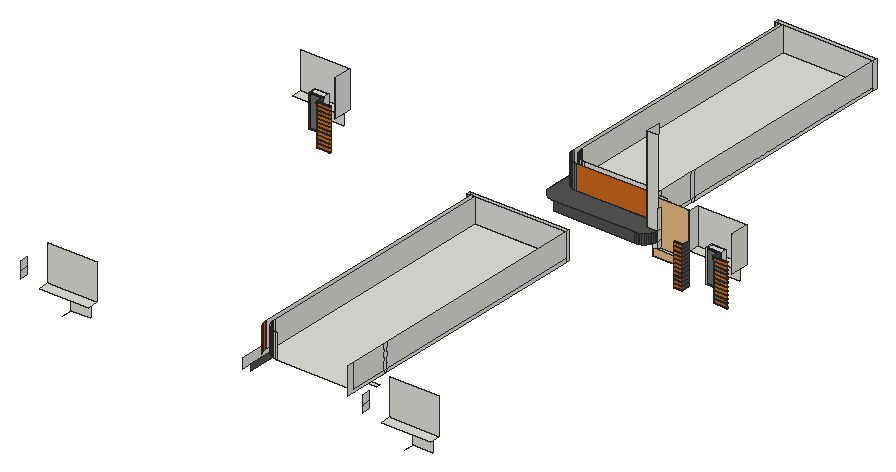
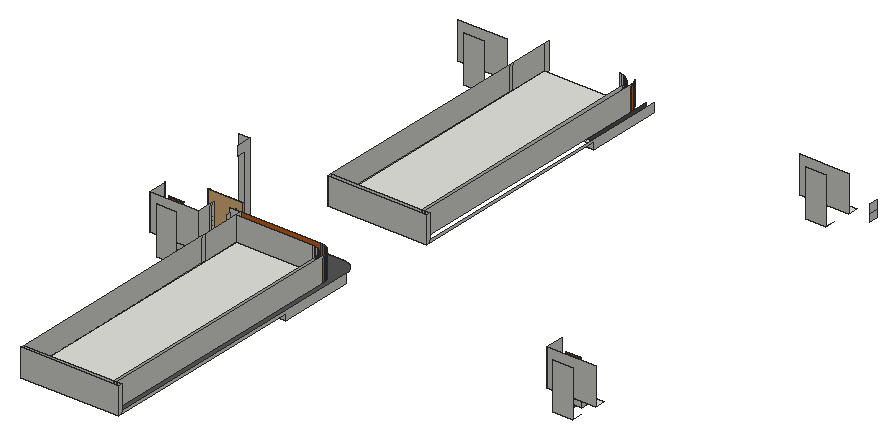
# SketchUp Ruby script. Lengths in inches.
U = 1.inch
M = Sketchup.active_model
def pt(a) = Geom::Point3d.new(a.map { |v| v * U })
def face(e, loops, mat)
  f = e.add_face(loops[0].map { |a| pt(a) })
  loops[1..].each { |l| e.add_face(l.map { |a| pt(a) }).erase! }
  f.material = f.back_material = mat if mat
  f
end
# faces: each face lists its corners as indices into pts; further lists are holes
def faces(e, pts, list, mat = nil) = list.each { |f| face(e, (f[0].is_a?(Array) ? f : [f]).map { |l| l.map { |i| pts[i] } }, mat) }
# xy, xz, yz: faces in a plane at the given z, y or x. An outline is a flat list of corners, or four numbers for a rectangle; further outlines are holes
def ring(l) = l.size == 4 ? [[l[0], l[1]], [l[2], l[1]], [l[2], l[3]], [l[0], l[3]]] : l.each_slice(2).to_a
def flat(e, list, mat, &to3) = list.each { |f| face(e, (f[0].is_a?(Array) ? f : [f]).map { |l| ring(l).map { |u, v| to3.(u, v) } }, mat) }
def xy(e, z, list, mat = nil) = flat(e, list, mat) { |x, y| [x, y, z] }
def xz(e, y, list, mat = nil) = flat(e, list, mat) { |x, z| [x, y, z] }
def yz(e, x, list, mat = nil) = flat(e, list, mat) { |y, z| [x, y, z] }
def lines(e, pts, list) = list.each { |a, b| e.add_line(pt(pts[a]), pt(pts[b])) }
# prism: a flat outline (further loops are holes) pulled along v
def prism(e, loops, v, mat = nil)
  f = face(e, loops, mat); d = Geom::Vector3d.new(v.map { |x| x * U })
  f.pushpull(f.normal.samedirection?(d) ? d.length : -d.length)
end
def box(e, o, s, mat = nil) = prism(e, [[o, [o[0] + s[0], o[1], o[2]], [o[0] + s[0], o[1] + s[1], o[2]], [o[0], o[1] + s[1], o[2]]]], [0, 0, s[2]], mat)
def at(x, y, z, deg = 0) = Geom::Transformation.translation(pt([x, y, z])) * Geom::Transformation.rotation(ORIGIN, Z_AXIS, deg.degrees)
def axes(o, x, y, z) = Geom::Transformation.new([*x, 0, *y, 0, *z, 0, *pt(o).to_a, 1])
def part(name) = M.definitions.add(name)
# library, detail: a bought-in or finely detailed component or shape, given as its bounding box
def library(name, o, s) = part(name).tap { |d| box(d.entities, o, s) }
def detail(e, o, s) = box(e.add_group.entities, o, s)
def put(e, d, t, mat = nil) = e.add_instance(d, t).tap { |i| i.material = mat if mat }
def group(e, t, mat = nil) = e.add_group.tap { |g| g.transformation = t; g.material = mat if mat }.entities
root = M.entities
M.materials.add("[0039_DarkOrange]").color = [219, 120, 0]
M.materials.add("[0041_Chocolate]").color = [210, 105, 30]
M.materials.add("[Color M06]").color = [84, 84, 84]
M.materials.add("[Translucent Glass Gray]").color = [0, 0, 0]
M.materials["[Translucent Glass Gray]"].alpha = 0.5
c1 = library("1",[3.97,34.78,0],[101.43,33.99,0.79])
xy(root,180.58,[[1550.98,971.36,1577.46,972.36],[2230.65,971.36,2246.03,972.36],[2305.61,971.36,2332.08,972.36]],"[0041_Chocolate]")
xy(root,182.6875,[[1550.98,971.36,1577.46,972.36],[2230.65,971.36,2246.03,972.36],[2305.61,971.36,2332.08,972.36]],"[0041_Chocolate]")
xy(root,187.64,[[1550.98,971.36,1577.46,972.36],[2230.65,971.36,2246.03,972.36],[2305.61,971.36,2332.08,972.36]],"[0041_Chocolate]")
xy(root,189.75,[[1550.98,971.36,1577.46,972.36],[2230.65,971.36,2246.03,972.36],[2305.61,971.36,2332.08,972.36]],"[0041_Chocolate]")
xy(root,194.7,[[1550.98,971.36,1577.46,972.36],[2230.65,971.36,2246.03,972.36],[2305.61,971.36,2332.08,972.36]],"[0041_Chocolate]")
xy(root,196.8125,[[1550.98,971.36,1577.46,972.36],[2305.61,971.36,2332.08,972.36]],"[0039_DarkOrange]")
xy(root,196.8125,[[2230.65,971.36,2246.03,972.36]],"[0041_Chocolate]")
xy(root,196.89,[[1523.64,986.55,1550.33,989.22],[2278.27,986.55,2304.96,989.22],[1523.64,990.13,1550.33,1001.8],[2278.27,990.13,2304.96,1001.8]])
xy(root,201.77,[[1550.98,971.36,1577.46,972.36],[2305.61,971.36,2332.08,972.36]],"[0039_DarkOrange]")
xy(root,201.77,[[2230.65,971.36,2246.03,972.36]],"[0041_Chocolate]")
xy(root,203.875,[[1550.98,971.36,1577.46,972.36],[2305.61,971.36,2332.08,972.36]],"[0039_DarkOrange]")
xy(root,203.875,[[2230.65,971.36,2246.03,972.36]],"[0041_Chocolate]")
xy(root,208.83,[[1550.98,971.36,1577.46,972.36],[2305.61,971.36,2332.08,972.36]],"[0039_DarkOrange]")
xy(root,208.83,[[2230.65,971.36,2246.03,972.36]],"[0041_Chocolate]")
xy(root,210.9375,[[1550.98,971.36,1577.46,972.36],[2305.61,971.36,2332.08,972.36]],"[0039_DarkOrange]")
xy(root,210.9375,[[2230.65,971.36,2246.03,972.36]],"[0041_Chocolate]")
xy(root,215.89,[[1550.98,971.36,1577.46,972.36],[2305.61,971.36,2332.08,972.36]],"[0039_DarkOrange]")
xy(root,215.89,[[2230.65,971.36,2246.03,972.36]],"[0041_Chocolate]")
xy(root,218,[[1550.98,971.36,1577.46,972.36],[2305.61,971.36,2332.08,972.36]],"[0039_DarkOrange]")
xy(root,218,[[2230.65,971.36,2246.03,972.36]],"[0041_Chocolate]")
xy(root,222.95,[[1550.98,971.36,1577.46,972.36],[2305.61,971.36,2332.08,972.36]],"[0039_DarkOrange]")
xy(root,222.95,[[2230.65,971.36,2246.03,972.36]],"[0041_Chocolate]")
xy(root,225.0625,[[1550.98,971.36,1577.46,972.36],[2305.61,971.36,2332.08,972.36]],"[0039_DarkOrange]")
xy(root,225.0625,[[2230.65,971.36,2246.03,972.36]],"[0041_Chocolate]")
xy(root,226.8,[[1547.71,317.3125,1640.52,337.5625],[2198.21,317.3125,2291.02,337.5625],[2181.03,983.34,2190.68,996.48],[2190.68,983.34,2230.65,1028.46],[1476.02,1008.21,1568.84,1028.46],
  [2230.65,1008.21,2323.46,1028.46]])
xy(root,227.53,[[2078.42,395.98,2125.61,403.17],[2110.86,1086.875,2158.05,1094.0625]])
xy(root,230.02,[[1550.98,971.36,1577.46,972.36],[2305.61,971.36,2332.08,972.36]],"[0039_DarkOrange]")
xy(root,230.02,[[2230.65,971.36,2246.03,972.36]],"[0041_Chocolate]")
xy(root,232.125,[[1550.98,971.36,1577.46,972.36],[2305.61,971.36,2332.08,972.36]],"[0039_DarkOrange]")
xy(root,232.125,[[2230.65,971.36,2246.03,972.36]],"[0041_Chocolate]")
xy(root,237.08,[[1550.98,971.36,1577.46,972.36],[2305.61,971.36,2332.08,972.36]],"[0039_DarkOrange]")
xy(root,237.08,[[2230.65,971.36,2246.03,972.36]],"[0041_Chocolate]")
xy(root,239.1875,[[1550.98,971.36,1577.46,972.36],[2230.65,971.36,2246.03,972.36],[2305.61,971.36,2332.08,972.36]],"[0041_Chocolate]")
xy(root,240.16,[[2166.32,969.24,2169.44,972.36],[2166.57,972.36,2167.81,972.44,2169.03,972.69,2169.44,972.82,2169.44,972.36],[2169.44,972.36,2169.44,972.82,2170.21,973.09,2171.33,973.64,2172.37,974.33,2173.31,975.15,2174.13,976.09,2174.82,977.13,2175.375,978.25,2175.77,979.43,2176.02,980.65,2176.1,981.89,2169.44,981.89,2169.44,983.34,2189.82,983.34,2189.82,981.89,2189.62,978.86,2189.02,975.875,2188.05,973,2187.73,972.36],[2187.73,972.36,2190.68,972.36,2190.68,981.89,2189.82,981.89,2189.62,978.86,2189.02,975.875,2188.05,973],[2169.44,972.82,2170.21,973.09,2171.33,973.64,2172.37,974.33,2173.31,975.15,2174.13,976.09,2174.82,977.13,2175.375,978.25,2175.77,979.43,2176.02,980.65,2176.1,981.89,2169.44,981.89],
  [2189.82,981.89,2190.68,983.34],[2169.44,983.34,2189.82,1003.71],[2189.82,983.34,2190.68,1003.71]])
xy(root,240.16,[[1949.9,333.33,1963.61,439.98],[2012.97,958.64,2012.97,972.36,2132.44,972.36,2132.44,969.24,2135.57,969.24,2135.57,972.36,2136.69,972.36,2136.69,969.24,2139.82,969.24,2139.82,972.36,2140.94,972.36,2140.94,969.24,2144.07,969.24,2144.07,972.36,2145.19,972.36,2145.19,969.24,2148.32,969.24,2148.32,972.36,2149.38,972.36,2149.38,969.24,2152.5,969.24,2152.5,972.36,2153.57,972.36,2153.57,969.24,2156.69,969.24,2156.69,972.36,2157.75,972.36,2157.75,969.24,2160.88,969.24,2160.88,972.36,2161.94,972.36,2161.94,969.24,2165.07,969.24,2165.07,972.36,2166.32,972.36,2166.32,969.24,2169.44,969.24,2169.44,972.36,2187.73,972.36,2186.7,970.27,2185.01,967.74,2183.01,965.45,2180.72,963.45,2178.19,961.76,2175.46,960.41,2172.58,959.4375,2169.6,958.84,2166.57,958.64],[1982.33,1024.22,1996.05,1130.875]],"[Color M06]")
xy(root,244.14,[[1550.98,971.36,1577.46,972.36],[2230.65,971.36,2246.03,972.36],[2305.61,971.36,2332.08,972.36]],"[0041_Chocolate]")
xy(root,246.25,[[1550.98,971.36,1577.46,972.36],[2230.65,971.36,2246.03,972.36],[2305.61,971.36,2332.08,972.36]],"[0041_Chocolate]")
xy(root,251.2,[[1550.98,971.36,1577.46,972.36],[2230.65,971.36,2246.03,972.36],[2305.61,971.36,2332.08,972.36]],"[0041_Chocolate]")
xy(root,252.47,[[[2066.68,395.98,2137,395.98,2137,403.17,2084.26,403.17,2084.26,439.98,2137,439.98,2137,830.91,1949.9,830.91,1949.9,439.98,2066.68,439.98],[1955.4,445.49,2131.5,825.41]],[2084.26,403.17,2137,439.98],[1949.9,830.91,2137,838.14],[2012.97,972.36,2010.76,972.5,2008.59,972.9375,2006.5,973.65,2004.51,974.63,2002.67,975.86,2001.01,977.32,1999.55,978.98,1998.32,980.82,1997.34,982.81,1996.625,984.9,1996.2,987.07,1996.05,989.28,1996.05,1130.875,2099.12,1130.875,2099.12,1086.875,2169.44,1086.875,2169.44,981.89,2176.1,981.89,2176.02,980.65,2175.77,979.43,2175.375,978.25,2174.82,977.13,2174.13,976.09,2173.31,975.15,2172.37,974.33,2171.33,973.64,2170.21,973.09,2169.03,972.69,2167.81,972.44,2166.57,972.36],[[2099.12,1086.875,2169.44,1086.875,2169.44,1094.0625,2116.69,1094.0625,2116.69,1130.875,2169.44,1130.875,2169.44,1521.81,1982.33,1521.81,1982.33,1130.875,2099.12,1130.875],[1987.84,1136.38,2163.94,1516.3]],
  [2116.69,1094.0625,2169.44,1130.875],[1982.33,1521.81,2169.44,1529.04]])
xy(root,253.3125,[[1550.98,971.36,1577.46,972.36],[2230.65,971.36,2246.03,972.36],[2305.61,971.36,2332.08,972.36]],"[0041_Chocolate]")
xy(root,258.13,[[1993.24,325.34,2137,325.34,2137,830.91,1965.22,830.91,1965.22,353.36,1965.46,349.7,1966.18,346.11,1967.36,342.64,1968.98,339.35,1971.01,336.3,1973.43,333.55,1976.1875,331.13,1979.23,329.09,1982.52,327.47,1985.99,326.29,1989.59,325.58],[2189.82,983.34,2190.68,1003.71],[2025.68,1016.23,2169.44,1016.23,2169.44,1521.81,1997.66,1521.81,1997.66,1044.25,1997.9,1040.6,1998.62,1037,1999.8,1033.53,2001.42,1030.24,2003.45,1027.2,2005.87,1024.44,2008.625,1022.02,2011.67,1019.99,2014.96,1018.37,2018.43,1017.1875,2022.02,1016.47]])
xy(root,258.13,[[2012.97,958.64,2166.57,958.64,2169.6,958.84,2172.58,959.4375,2175.46,960.41,2178.19,961.76,2180.72,963.45,2183.01,965.45,2185.01,967.74,2186.7,970.27,2188.05,973,2189.02,975.875,2189.62,978.86,2189.82,981.89,2189.82,1003.71,2019.9375,1003.71,2016.14,1003.96,2012.42,1004.7,2008.82,1005.92,2005.41,1007.6,2002.25,1009.71,1999.39,1012.22,1996.88,1015.08,1996.11,1016.23,1994.77,1018.24,1993.09,1021.65,1991.87,1025.25,1991.125,1028.97,1990.88,1032.77,1990.88,1521.81,1982.33,1521.81,1982.33,989.28,1982.6,985.28,1983.38,981.35,1984.67,977.56,1986.4375,973.96,1988.67,970.63,1991.31,967.62,1994.32,964.98,1997.65,962.75,2001.25,960.98,2005.04,959.6875,2008.97,958.91]],"[Color M06]")
xy(root,258.27,[[1523.64,986.55,1550.33,989.22],[2278.27,986.55,2304.96,989.22],[1523.64,989.22,1550.33,990.13],[2278.27,989.22,2304.96,990.13],[1523.64,990.13,1550.33,1001.8],
  [2278.27,990.13,2304.96,1001.8]])
xy(root,258.27,[[1550.33,971.36,1577.46,972.36],[2230.65,971.36,2246.69,972.36],[2304.96,971.36,2332.08,972.36]],"[0041_Chocolate]")
xz(root,337.5625,[[1547.71,226.8,1640.52,295.72],[2198.21,226.8,2291.02,295.72]])
xz(root,341.65,[[1588.08,192.35,1624.95,281.26],[2238.58,192.35,2275.45,281.26]])
xz(root,439.98,[[1949.9,240.16,1963.61,252.47]])
xz(root,830.91,[[1949.9,252.47,1949.9,258.13,1958.44,258.13,1958.44,304.25,1965.22,304.25,1965.22,258.13,2137,258.13,2137,252.47],[1949.9,258.13,1958.44,304.25],[1965.22,258.13,2137,304.25]])
xz(root,838.14,[[1949.9,252.47,2137,304.25]])
xz(root,958.64,[[2012.97,240.16,2166.57,258.13]],"[Color M06]")
xz(root,971.36,[[1550.98,196.8125,1577.46,201.77],[2305.61,196.8125,2332.08,201.77],[1550.98,203.875,1577.46,208.83],[2305.61,203.875,2332.08,208.83],[1550.98,210.9375,1577.46,215.89],
  [2305.61,210.9375,2332.08,215.89],[1550.98,218,1577.46,222.95],[2305.61,218,2332.08,222.95],[1550.98,225.0625,1577.46,230.02],[2305.61,225.0625,2332.08,230.02],
  [1550.98,232.125,1577.46,237.08],[2305.61,232.125,2332.08,237.08]],"[0039_DarkOrange]")
xz(root,971.36,[[1550.98,182.6875,1577.46,187.64],[2230.65,182.6875,2246.03,187.64],[2305.61,182.6875,2332.08,187.64],[1550.98,189.75,1577.46,194.7],[2230.65,189.75,2246.03,194.7],
  [2305.61,189.75,2332.08,194.7],[2230.65,196.8125,2246.03,201.77],[2230.65,203.875,2246.03,208.83],[2230.65,210.9375,2246.03,215.89],[2230.65,218,2246.03,222.95],
  [2230.65,225.0625,2246.03,230.02],[2230.65,232.125,2246.03,237.08],[1550.98,239.1875,1577.46,244.14],[2230.65,239.1875,2246.03,244.14],[2305.61,239.1875,2332.08,244.14],
  [1550.98,246.25,1577.46,251.2],[2230.65,246.25,2246.03,251.2],[2305.61,246.25,2332.08,251.2],[1550.98,253.3125,1577.46,253.3125,1577.46,258.27,1550.33,258.27],[2230.65,253.3125,2246.03,253.3125,2246.69,258.27,2230.65,258.27],
  [2305.61,253.3125,2332.08,253.3125,2332.08,258.27,2304.96,258.27]],"[0041_Chocolate]")
xz(root,972.36,[[2012.97,240.16,2166.57,252.47]])
xz(root,972.36,[[1550.98,201.77,1577.46,203.875],[2305.61,201.77,2332.08,203.875],[1550.98,208.83,1577.46,210.9375],[2305.61,208.83,2332.08,210.9375],[1550.98,215.89,1577.46,218],
  [2305.61,215.89,2332.08,218],[1550.98,222.95,1577.46,225.0625],[2305.61,222.95,2332.08,225.0625],[1550.98,230.02,1577.46,232.125],[2305.61,230.02,2332.08,232.125],
  [1550.98,237.08,1577.46,239.1875],[2305.61,237.08,2332.08,239.1875]],"[0039_DarkOrange]")
xz(root,972.36,[[1550.98,180.58,1577.46,182.6875],[2230.65,180.58,2246.03,182.6875],[2305.61,180.58,2332.08,182.6875],[1550.98,187.64,1577.46,189.75],[2230.65,187.64,2246.03,189.75],
  [2305.61,187.64,2332.08,189.75],[1550.98,194.7,1577.46,196.8125],[2230.65,194.7,2246.03,196.8125],[2305.61,194.7,2332.08,196.8125],[2230.65,201.77,2246.03,203.875],
  [2230.65,208.83,2246.03,210.9375],[2230.65,215.89,2246.03,218],[2230.65,222.95,2246.03,225.0625],[2230.65,230.02,2246.03,232.125],[2230.65,237.08,2246.03,239.1875],
  [1550.98,244.14,1577.46,246.25],[2230.65,244.14,2246.03,246.25],[2305.61,244.14,2332.08,246.25],[1550.98,251.2,1577.46,253.3125],[2230.65,251.2,2246.03,253.3125],
  [2305.61,251.2,2332.08,253.3125],[1550.33,258.27,1577.46,258.27,1577.46,260.375,1550.05,260.375],[2230.65,258.27,2246.69,258.27,2246.96,260.375,2230.65,260.375],[2304.96,258.27,2332.08,258.27,2332.08,260.375,2304.68,260.375]],"[0041_Chocolate]")
xz(root,981.89,[[2169.44,240.16,2176.1,252.47]])
xz(root,983.34,[[2181.03,226.8,2190.68,240.16],[2169.44,240.16,2189.82,240.16,2189.82,258.13,2190.68,258.13,2190.68,421.25,2169.44,421.25],[2189.82,240.16,2190.68,258.13]])
xz(root,989.22,[[1523.64,196.89,1550.33,258.27],[2278.27,196.89,2304.96,258.27]],"[Translucent Glass Gray]")
xz(root,990.13,[[1523.64,196.89,1550.33,258.27],[2278.27,196.89,2304.96,258.27]])
xz(root,1001.8,[[1523.64,196.89,1550.33,258.27],[2278.27,196.89,2304.96,258.27]])
xz(root,1003.71,[[2169.44,240.16,2189.82,258.13],[2189.82,240.16,2190.68,258.13],[2169.44,258.13,2190.68,304.25]])
xz(root,1003.71,[[2019.9375,258.13,2169.44,304.25]],"[0041_Chocolate]")
xz(root,1016.23,[[2025.68,258.13,2169.44,304.25]])
xz(root,1028.46,[[1476.02,226.8,1568.84,295.72],[2230.65,226.8,2323.46,295.72]])
xz(root,1032.54,[[1516.4,192.35,1553.26,281.26],[2271.02,192.35,2307.88,281.26]])
xz(root,1130.875,[[1982.33,240.16,1996.05,252.47]])
xz(root,1521.81,[[1982.33,252.47,1982.33,258.13,1990.88,258.13,1990.88,304.25,1997.66,304.25,1997.66,258.13,2169.44,258.13,2169.44,252.47],[1982.33,258.13,1990.88,304.25],[1997.66,258.13,2169.44,304.25]])
xz(root,1529.04,[[1982.33,252.47,2169.44,304.25]])
yz(root,1507.74,[[321.34,226.8,337.5625,240.16],[321.34,240.16,337.5625,258.13]])
yz(root,1523.64,[[986.55,196.89,989.22,258.27],[990.13,196.89,1001.8,258.27]])
yz(root,1550.33,[[986.55,196.89,989.22,258.27],[990.13,196.89,1001.8,258.27]])
yz(root,1550.98,[[972.36,180.58,986.55,182.6875],[971.36,182.6875,986.55,187.64],[972.36,187.64,986.55,189.75],[971.36,189.75,986.55,194.7],[972.36,194.7,986.55,196.8125],
  [971.36,196.8125,986.55,201.77],[972.36,201.77,986.55,203.875],[971.36,203.875,986.55,208.83],[972.36,208.83,986.55,210.9375],[971.36,210.9375,986.55,215.89],
  [972.36,215.89,986.55,218],[971.36,218,986.55,222.95],[972.36,222.95,986.55,225.0625],[971.36,225.0625,986.55,230.02],[972.36,230.02,986.55,232.125],
  [971.36,232.125,986.55,237.08],[972.36,237.08,986.55,239.1875],[971.36,239.1875,986.55,244.14],[972.36,244.14,986.55,246.25],[971.36,246.25,986.55,251.2],
  [972.36,251.2,986.55,253.3125]],"[Color M06]")
yz(root,1568.84,[[992.96,226.8,993.35,295.72],[993.35,226.8,1028.46,295.72]])
yz(root,1949.9,[[298.39,240.16,298.39,258.13,830.91,258.13,830.91,252.47,439.98,252.47,439.98,240.16],[830.91,252.47,838.14,304.25]])
yz(root,1958.44,[[341.87,258.13,830.91,304.25]])
yz(root,1963.61,[[298.39,240.16,439.98,252.47]],"[Color M06]")
yz(root,1965.22,[[353.36,258.13,830.91,304.25]])
yz(root,1982.33,[[989.28,240.16,989.28,258.13,1521.81,258.13,1521.81,252.47,1130.875,252.47,1130.875,240.16],[1521.81,252.47,1529.04,304.25]])
yz(root,1990.88,[[1032.77,258.13,1521.81,304.25]])
yz(root,1996.05,[[989.28,240.16,1130.875,252.47]],"[Color M06]")
yz(root,1997.66,[[1044.25,258.13,1521.81,304.25]])
yz(root,2137,[[312.8125,252.47,397.86,252.47,397.86,258.13,325.34,258.13,325.34,304.25,312.8125,304.25],[397.86,252.47,406.38,258.13],[406.38,252.47,830.91,258.13],[830.91,252.47,838.14,304.25],[325.34,258.13,397.86,304.25],
  [397.86,258.13,406.38,304.25],[406.38,258.13,830.91,304.25]])
yz(root,2158.24,[[321.34,226.8,337.5625,240.16],[321.34,240.16,337.5625,258.13]])
yz(root,2169.44,[[981.89,240.16,983.34,252.47],[983.34,240.16,996.48,252.47],[996.48,240.16,1003.71,252.47],[983.34,252.47,983.34,421.25,1012.23,421.25,1012.23,402.64,996.48,402.64,996.48,252.47],[1003.71,252.47,1088.75,252.47,1088.75,258.13,1016.23,258.13,1016.23,304.25,1003.71,304.25],
  [1088.75,252.47,1097.28,258.13],[1097.28,252.47,1521.81,258.13],[1521.81,252.47,1529.04,304.25],[1016.23,258.13,1088.75,304.25],[1088.75,258.13,1097.28,304.25],
  [1097.28,258.13,1521.81,304.25]])
yz(root,2189.82,[[981.89,240.16,983.34,258.13],[983.34,240.16,1003.71,258.13]])
yz(root,2190.68,[[983.34,226.8,996.48,240.16],[996.48,226.8,1012.23,240.16],[1012.23,226.8,1028.46,240.16],[983.34,240.16,996.48,258.13],[1003.71,240.16,1012.23,258.13],
  [1012.23,240.16,1028.46,258.13],[983.34,258.13,996.48,295.72],[996.48,258.13,1003.71,295.72],[1003.71,258.13,1012.23,295.72]])
yz(root,2230.65,[[992.96,226.8,993.35,295.72],[993.35,226.8,996.48,295.72],[996.48,226.8,1001.16,295.72],[1001.16,226.8,1028.46,295.72]])
yz(root,2246.03,[[972.36,180.58,986.55,182.6875],[971.36,182.6875,986.55,187.64],[972.36,187.64,986.55,189.75],[971.36,189.75,986.55,194.7],[972.36,194.7,986.55,196.8125],
  [971.36,196.8125,986.55,201.77],[972.36,201.77,986.55,203.875],[971.36,203.875,986.55,208.83],[972.36,208.83,986.55,210.9375],[971.36,210.9375,986.55,215.89],
  [972.36,215.89,986.55,218],[971.36,218,986.55,222.95],[972.36,222.95,986.55,225.0625],[971.36,225.0625,986.55,230.02],[972.36,230.02,986.55,232.125],
  [971.36,232.125,986.55,237.08],[972.36,237.08,986.55,239.1875],[971.36,239.1875,986.55,244.14],[972.36,244.14,986.55,246.25],[971.36,246.25,986.55,251.2],
  [972.36,251.2,986.55,253.3125]],"[Color M06]")
yz(root,2278.27,[[986.55,196.89,989.22,258.27],[990.13,196.89,1001.8,258.27]])
yz(root,2304.96,[[986.55,196.89,989.22,258.27],[990.13,196.89,1001.8,258.27]])
yz(root,2305.61,[[972.36,180.58,986.55,182.6875],[971.36,182.6875,986.55,187.64],[972.36,187.64,986.55,189.75],[971.36,189.75,986.55,194.7],[972.36,194.7,986.55,196.8125],
  [971.36,196.8125,986.55,201.77],[972.36,201.77,986.55,203.875],[971.36,203.875,986.55,208.83],[972.36,208.83,986.55,210.9375],[971.36,210.9375,986.55,215.89],
  [972.36,215.89,986.55,218],[971.36,218,986.55,222.95],[972.36,222.95,986.55,225.0625],[971.36,225.0625,986.55,230.02],[972.36,230.02,986.55,232.125],
  [971.36,232.125,986.55,237.08],[972.36,237.08,986.55,239.1875],[971.36,239.1875,986.55,244.14],[972.36,244.14,986.55,246.25],[971.36,246.25,986.55,251.2],
  [972.36,251.2,986.55,253.3125]],"[Color M06]")
yz(root,2323.46,[[992.96,226.8,993.35,295.72],[993.35,226.8,1028.46,295.72]])
p = [[2169.6,958.84,258.13],[2166.57,958.64,258.13],[2166.57,958.64,240.16],[2169.6,958.84,240.16],[2172.58,959.4375,258.13],[2172.58,959.4375,240.16],
  [2175.46,960.41,258.13],[2175.46,960.41,240.16],[2178.19,961.76,258.13],[2178.19,961.76,240.16],[2180.72,963.45,258.13],[2180.72,963.45,240.16],
  [2183.01,965.45,258.13],[2183.01,965.45,240.16],[2185.01,967.74,258.13],[2185.01,967.74,240.16],[2186.7,970.27,258.13],[2186.7,970.27,240.16],
  [2188.05,973,258.13],[2187.73,972.36,240.16],[2188.05,973,240.16],[2166.57,972.36,252.47],[2167.81,972.44,252.47],[2167.81,972.44,240.16],
  [2166.57,972.36,240.16],[2169.03,972.69,252.47],[2169.03,972.69,240.16],[2170.21,973.09,252.47],[2170.21,973.09,240.16],[2169.44,972.82,240.16],
  [2189.02,975.875,258.13],[2189.02,975.875,240.16],[2171.33,973.64,252.47],[2171.33,973.64,240.16],[2172.37,974.33,252.47],[2172.37,974.33,240.16],
  [2173.31,975.15,252.47],[2173.31,975.15,240.16],[2174.13,976.09,252.47],[2174.13,976.09,240.16],[2189.62,978.86,258.13],[2189.62,978.86,240.16],
  [2174.82,977.13,252.47],[2174.82,977.13,240.16],[2175.375,978.25,252.47],[2175.375,978.25,240.16],[2175.77,979.43,252.47],[2175.77,979.43,240.16],
  [2189.82,981.89,258.13],[2189.82,981.89,240.16],[2176.02,980.65,252.47],[2176.02,980.65,240.16],[2176.1,981.89,252.47],[2176.1,981.89,240.16],
  [1550.98,986.55,253.3125],[1550.98,972.36,253.3125],[1550.98,971.36,253.3125],[1550.33,971.36,258.27],[1550.33,972.36,258.27],[1550.33,986.55,258.27],
  [2246.69,986.55,258.27],[2246.69,972.36,258.27],[2246.69,971.36,258.27],[2246.03,971.36,253.3125],[2246.03,972.36,253.3125],[2246.03,986.55,253.3125],
  [2305.61,986.55,253.3125],[2305.61,972.36,253.3125],[2305.61,971.36,253.3125],[2304.96,971.36,258.27],[2304.96,972.36,258.27],[2304.96,986.55,258.27],
  [1962.33,327.34,258.13],[1963.67,325.34,258.13],[1963.67,325.34,304.25],[1962.33,327.34,304.25],[1993.24,325.34,258.13],[1989.59,325.58,258.13],
  [1989.59,325.58,304.25],[1993.24,325.34,304.25],[1985.99,326.29,258.13],[1985.99,326.29,304.25],[1982.52,327.47,258.13],[1982.52,327.47,304.25],
  [1960.65,330.75,258.13],[1960.65,330.75,304.25],[1979.23,329.09,258.13],[1979.23,329.09,304.25],[1976.1875,331.13,258.13],[1976.1875,331.13,304.25],
  [1959.43,334.35,258.13],[1959.43,334.35,304.25],[1973.43,333.55,258.13],[1973.43,333.55,304.25],[1971.01,336.3,258.13],[1971.01,336.3,304.25],
  [1958.6875,338.08,258.13],[1958.6875,338.08,304.25],[1968.98,339.35,258.13],[1968.98,339.35,304.25],[1958.44,341.87,258.13],[1958.44,341.87,304.25],
  [1967.36,342.64,258.13],[1967.36,342.64,304.25],[1966.18,346.11,258.13],[1966.18,346.11,304.25],[1965.46,349.7,258.13],[1965.46,349.7,304.25],
  [1965.22,353.36,258.13],[1965.22,353.36,304.25],[2016.14,1003.96,258.13],[2019.9375,1003.71,258.13],[2019.9375,1003.71,304.25],[2016.14,1003.96,304.25],
  [2012.42,1004.7,258.13],[2012.42,1004.7,304.25],[2008.82,1005.92,258.13],[2008.82,1005.92,304.25],[2005.41,1007.6,258.13],[2005.41,1007.6,304.25],
  [2002.25,1009.71,258.13],[2002.25,1009.71,304.25],[1999.39,1012.22,258.13],[1999.39,1012.22,304.25],[1996.88,1015.08,258.13],[1997.66,1014.1875,304.25],
  [1996.88,1015.08,304.25],[1996.11,1016.23,258.13],[1996.11,1016.23,304.25],[1994.77,1018.24,258.13],[1994.77,1018.24,304.25],[2025.68,1016.23,258.13],
  [2022.02,1016.47,258.13],[2022.02,1016.47,304.25],[2025.68,1016.23,304.25],[2018.43,1017.1875,258.13],[2018.43,1017.1875,304.25],[2014.96,1018.37,258.13],
  [2014.96,1018.37,304.25],[1993.09,1021.65,258.13],[1993.09,1021.65,304.25],[2011.67,1019.99,258.13],[2011.67,1019.99,304.25],[2008.625,1022.02,258.13],
  [2008.625,1022.02,304.25],[1991.87,1025.25,258.13],[1991.87,1025.25,304.25],[2005.87,1024.44,258.13],[2005.87,1024.44,304.25],[2003.45,1027.2,258.13],
  [2003.45,1027.2,304.25],[1991.125,1028.97,258.13],[1991.125,1028.97,304.25],[2001.42,1030.24,258.13],[2001.42,1030.24,304.25],[1990.88,1032.77,258.13],
  [1990.88,1032.77,304.25],[1999.8,1033.53,258.13],[1999.8,1033.53,304.25],[1998.62,1037,258.13],[1998.62,1037,304.25],[1997.9,1040.6,258.13],
  [1997.9,1040.6,304.25],[1997.66,1044.25,258.13],[1997.66,1044.25,304.25],[1550.05,972.36,260.375],[1550.05,986.55,260.375],[2246.96,972.36,260.375],
  [2246.96,986.55,260.375],[2304.68,972.36,260.375],[2304.68,986.55,260.375],[1588.08,321.34,192.35],[1588.08,341.65,192.35],[2238.58,321.34,192.35],
  [2238.58,341.65,192.35],[1516.4,1012.23,192.35],[1516.4,1032.54,192.35],[2271.02,1012.23,192.35],[2271.02,1032.54,192.35]]
faces(root,p,[[0,1,2,3],[4,0,3,5],[6,4,5,7],[8,6,7,9],[10,8,9,11],[12,10,11,13],[14,12,13,15],[16,14,15,17],
  [18,16,17,19,20],[30,18,20,31],[40,30,31,41],[48,40,41,49],[54,55,56,57,58,59],[60,61,62,63,64,65],[66,67,68,69,70,71],[58,165,166,59],
  [167,61,60,168],[70,169,170,71]],"[Color M06]")
faces(root,p,[[21,22,23,24],[22,25,26,23],[25,27,28,29,26],[27,32,33,28],[32,34,35,33],[34,36,37,35],[36,38,39,37],[38,42,43,39],
  [42,44,45,43],[44,46,47,45],[46,50,51,47],[50,52,53,51],[76,77,78,79],[77,80,81,78],[80,82,83,81],[82,86,87,83],
  [86,88,89,87],[88,92,93,89],[92,94,95,93],[94,98,99,95],[98,102,103,99],[102,104,105,103],[104,106,107,105],[106,108,109,107],
  [131,132,133,134],[132,135,136,133],[135,137,138,136],[137,141,142,138],[141,143,144,142],[143,147,148,144],[147,149,150,148],[149,153,154,150],
  [153,157,158,154],[157,159,160,158],[159,161,162,160],[161,163,164,162]])
faces(root,p,[[72,73,74,75],[84,72,75,85],[90,84,85,91],[96,90,91,97],[100,96,97,101],[110,111,112,113],[114,110,113,115],[116,114,115,117],
  [118,116,117,119],[120,118,119,121],[122,120,121,123],[124,122,123,125,126],[127,124,126,128],[129,127,128,130],[139,129,130,140],[145,139,140,146],
  [151,145,146,152],[155,151,152,156]],"[0041_Chocolate]")
lines(root,p,[[171,172],[173,174],[175,176],[177,178]])
put(root,c1,axes([2314.31,990.33,204.87],[0,0,1],[-2,0,0],[0,-1,0]))
